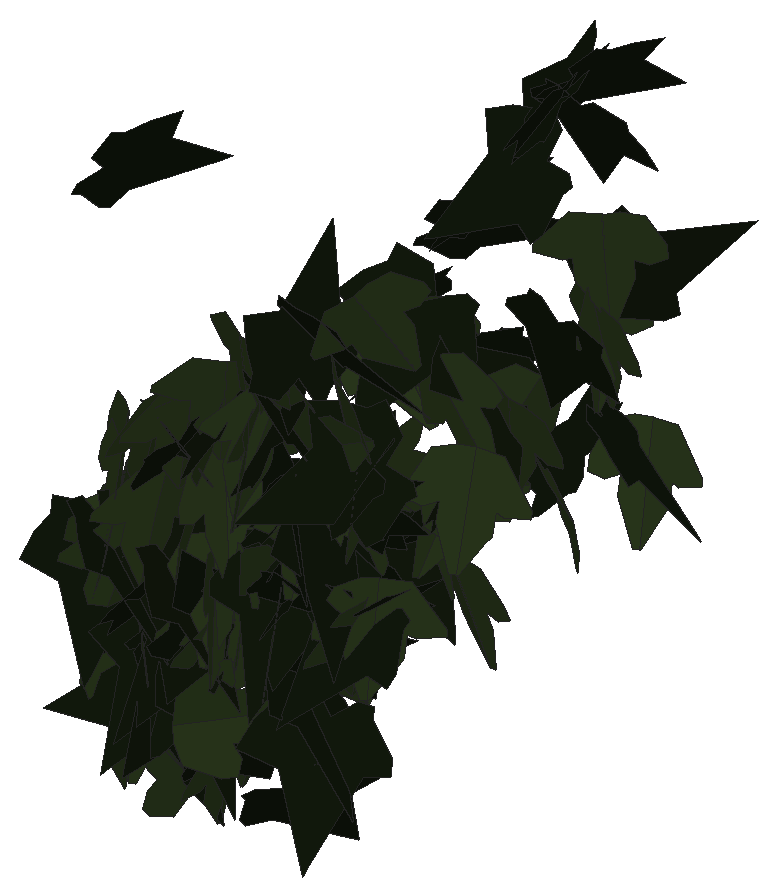
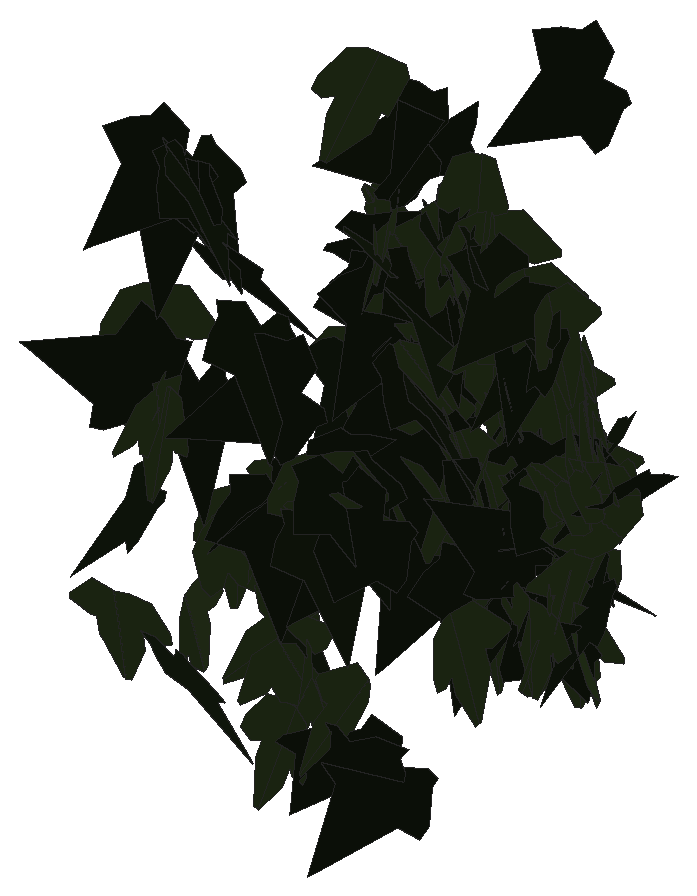
# SketchUp Ruby script. Lengths in inches.
U = 1.inch
M = Sketchup.active_model
def pt(a) = Geom::Point3d.new(a.map { |v| v * U })
def face(e, loops, mat)
  f = e.add_face(loops[0].map { |a| pt(a) })
  loops[1..].each { |l| e.add_face(l.map { |a| pt(a) }).erase! }
  f.material = f.back_material = mat if mat
  f
end
# faces: each face lists its corners as indices into pts; further lists are holes
def faces(e, pts, list, mat = nil) = list.each { |f| face(e, (f[0].is_a?(Array) ? f : [f]).map { |l| l.map { |i| pts[i] } }, mat) }
# xy, xz, yz: faces in a plane at the given z, y or x. An outline is a flat list of corners, or four numbers for a rectangle; further outlines are holes
def ring(l) = l.size == 4 ? [[l[0], l[1]], [l[2], l[1]], [l[2], l[3]], [l[0], l[3]]] : l.each_slice(2).to_a
def flat(e, list, mat, &to3) = list.each { |f| face(e, (f[0].is_a?(Array) ? f : [f]).map { |l| ring(l).map { |u, v| to3.(u, v) } }, mat) }
def xy(e, z, list, mat = nil) = flat(e, list, mat) { |x, y| [x, y, z] }
def xz(e, y, list, mat = nil) = flat(e, list, mat) { |x, z| [x, y, z] }
def yz(e, x, list, mat = nil) = flat(e, list, mat) { |y, z| [x, y, z] }
def lines(e, pts, list) = list.each { |a, b| e.add_line(pt(pts[a]), pt(pts[b])) }
# prism: a flat outline (further loops are holes) pulled along v
def prism(e, loops, v, mat = nil)
  f = face(e, loops, mat); d = Geom::Vector3d.new(v.map { |x| x * U })
  f.pushpull(f.normal.samedirection?(d) ? d.length : -d.length)
end
def box(e, o, s, mat = nil) = prism(e, [[o, [o[0] + s[0], o[1], o[2]], [o[0] + s[0], o[1] + s[1], o[2]], [o[0], o[1] + s[1], o[2]]]], [0, 0, s[2]], mat)
def at(x, y, z, deg = 0) = Geom::Transformation.translation(pt([x, y, z])) * Geom::Transformation.rotation(ORIGIN, Z_AXIS, deg.degrees)
def axes(o, x, y, z) = Geom::Transformation.new([*x, 0, *y, 0, *z, 0, *pt(o).to_a, 1])
def part(name) = M.definitions.add(name)
# library, detail: a bought-in or finely detailed component or shape, given as its bounding box
def library(name, o, s) = part(name).tap { |d| box(d.entities, o, s) }
def detail(e, o, s) = box(e.add_group.entities, o, s)
def put(e, d, t, mat = nil) = e.add_instance(d, t).tap { |i| i.material = mat if mat }
def group(e, t, mat = nil) = e.add_group.tap { |g| g.transformation = t; g.material = mat if mat }.entities
root = M.entities
M.materials.add("efeu1").color = [18, 25, 13]
M.materials.add("efeu2").color = [43, 57, 29]
c1 = part("ivyleaf_10")
p = [[0,0.5,-0.03],[-0.0625,2.02,-0.43],[-0.19,2.01,-0.46],[-0.54,1.05,-0.29],[-0.52,0.625,-0.18],[-0.83,0.76,-0.28],
  [-1.16,0.64,-0.33],[-1.15,0.33,-0.24],[-0.77,-0.39,0.02],[-0.3,-0.51,0.16],[0.04,-0.48,0.23],[-0.02,2.01,-0.4375],
  [-0.06,2.01,-0.43],[0.04,-0.49,0.23],[0.67,-0.49,0.14],[1.38,0.36,-0.2],[1.375,0.51,-0.24],[0.81,0.65,-0.19],
  [0.62,0.59,-0.15],[0.6,1.09,-0.28],[0.5,1.23,-0.31]]
faces(c1.entities,p,[[0,1,2,3,4,5,6,7,8,9,10],[11,12,0,13,14,15,16,17,18,19,20]],"efeu2")
c2 = part("ivyleaf_9")
p = [[1.54,2.16,1.25],[1.36,2.04,1.19],[-0.21,0.99,0.68],[-0.71,1.11,0.82],[-0.85,0.86,0.67],[-0.8,0.17,0.21],
  [-0.9,-0.01,0.1],[-0.67,-0.16,-0.02],[-0.08,-0.08,-0.05],[-0.03,-0.6,-0.4],[0.65,-0.88,-0.66],[0.83,-0.6,-0.49],
  [1.29,-0.42,-0.43],[1.8125,-0.07,-0.26],[1.21,0.44,0.15]]
faces(c2.entities,p,[[0,1,2,3,4,5,6,7,8,9,10,11,12,13,14]],"efeu1")
put(root,c1,axes([41.9,223.25,236.34],[-0.14655,-0.46971,0.08886],[0.0345,-0.10309,-0.48804],[0.47679,-0.13692,0.06263]))
put(root,c1,axes([43.12,223.04,238.36],[-0.46033,0.12611,0.14896],[-0.14145,0.04738,-0.47723],[-0.13448,-0.48151,-0.00795]))
put(root,c1,axes([43.13,223.35,237.54],[-0.13883,-0.43112,0.21181],[0.04974,-0.2322,-0.44001],[0.47776,-0.1011,0.10736]))
put(root,c2,axes([43.88,223.33,234.49],[-0.31378,-0.34921,-0.17204],[0.11314,0.12963,-0.46946],[0.37248,-0.33355,-0.00233]))
put(root,c1,axes([41.27,223.24,235.78],[0.33453,-0.37126,0.0158],[0.02306,-0.00048,-0.49947],[0.37088,0.33491,0.0168]))
put(root,c2,axes([44.39,223.45,237.38],[-0.39107,-0.1524,0.27174],[-0.23964,-0.13155,-0.41865],[0.1991,-0.45768,0.02985]))
put(root,c2,axes([42.32,223.33,235.05],[-0.4867,-0.03334,-0.1096],[0.11067,-0.0132,-0.48742],[0.02961,-0.49871,0.02023]))
put(root,c2,axes([43.23,223.33,237.06],[-0.08331,-0.00209,-0.49301],[0.49276,-0.01636,-0.0832],[-0.01578,-0.49973,0.00479]))
put(root,c1,axes([42.57,223.3125,235.58],[-0.09073,0.40705,-0.27582],[0.05377,-0.27058,-0.41701],[-0.48875,-0.10533,0.00532]))
put(root,c2,axes([41.67,222.79,239.95],[0.25473,0.28777,0.31984],[0.21646,0.23551,-0.38429],[-0.37183,0.33425,-0.0046]))
put(root,c2,axes([43.83,223.43,236.4375],[0.06562,-0.48821,0.08567],[-0.0004,-0.08647,-0.49247],[0.49567,0.06457,-0.01174]))
put(root,c2,axes([43.4,223.39,235.9],[-0.38034,-0.27863,-0.16646],[0.1632,0.05748,-0.46911],[0.28055,-0.41117,0.04722]))
put(root,c1,axes([42.75,223.2,237.87],[-0.37516,-0.32831,0.03826],[-0.03439,-0.01878,-0.49846],[0.32874,-0.37664,-0.00849]))
put(root,c2,axes([41.2,223.29,235.71],[0.29546,-0.40334,-0.00453],[0.00177,0.00691,-0.49995],[0.40336,0.29542,0.00551]))
put(root,c1,axes([42.85,223.45,237.29],[0.25653,-0.28307,0.32259],[0.2162,-0.23943,-0.38201],[0.37075,0.33548,-0.00045]))
put(root,c2,axes([42.14,223.29,234.29],[-0.42513,0.12072,0.23386],[-0.24322,-0.01049,-0.43673],[-0.10054,-0.4851,0.06764]))
put(root,c1,axes([41.86,223.26,237.22],[0.04929,-0.49756,0.00001],[-0.00013,-0.00003,-0.5],[0.49756,0.04929,-0.00013]))
put(root,c1,axes([42.54,223.28,235.76],[0.49119,-0.06142,0.07044],[0.06923,-0.01408,-0.49498],[0.06278,0.49601,-0.00533]))
put(root,c2,axes([44.35,223.38,235.83],[-0.49168,-0.07529,-0.05078],[0.05089,0.00312,-0.49739],[0.07521,-0.49429,0.00459]))
put(root,c1,axes([44.15,223.48,237.24],[-0.09405,0.23419,-0.43163],[0.11552,-0.4166,-0.2512],[-0.47729,-0.14698,0.02426]))
put(root,c2,axes([41.78,223.6,234.07],[0.1439,-0.14496,-0.45638],[0.32512,-0.32029,0.20424],[-0.35156,-0.35553,0.00208]))
put(root,c2,axes([43.2,223.18,237.88],[0.4379,-0.23619,-0.04961],[-0.04004,0.03024,-0.49748],[0.23799,0.43966,0.00757]))
put(root,c1,axes([42.23,223.27,237.38],[-0.15829,-0.47427,-0.0041],[0.01044,0.00084,-0.49989],[0.47417,-0.15834,0.00964]))
put(root,c2,axes([42.84,223.1,237.58],[-0.2834,0.40684,0.06454],[-0.0429,0.04876,-0.49576],[-0.40969,-0.28653,0.00726]))
put(root,c2,axes([41.94,223.56,234.54],[-0.30019,-0.38956,0.09017],[-0.05344,-0.07266,-0.4918],[0.39627,-0.3049,0.00199]))
put(root,c1,axes([42.6875,222.89,234.24],[-0.00004,0.01216,0.49985],[0.131,0.48239,-0.01172],[-0.48253,0.13096,-0.00323]))
put(root,c2,axes([42.04,223.35,235.46],[0.2615,-0.42615,-0.00415],[0.0243,0.01977,-0.49902],[0.42547,0.26078,0.03105]))
put(root,c1,axes([41.32,223.34,236.53],[0.33725,-0.36605,0.04761],[0.06246,-0.00698,-0.49603],[0.36381,0.34053,0.04102]))
put(root,c1,axes([41.43,223.4,235.5625],[-0.17036,-0.44687,0.14588],[-0.01752,-0.14903,-0.47695],[0.46976,-0.16762,0.03512]))
put(root,c2,axes([43.49,223.41,234.8],[0.23339,-0.44121,0.02939],[0.02254,-0.02132,-0.49904],[0.44161,0.23426,0.00994]))
put(root,c2,axes([40.99,223.52,235.39],[-0.08743,-0.49224,0.00783],[0.00955,-0.00964,-0.49982],[0.4922,-0.08724,0.01109]))
put(root,c2,axes([43.65,223.26,238.7],[0.42423,-0.16786,0.20457],[0.20345,-0.04027,-0.45496],[0.16922,0.46925,0.03413]))
put(root,c1,axes([44.27,223.31,235.78],[-0.02645,-0.49573,-0.0596],[0.00143,0.05961,-0.49643],[0.4993,-0.02643,-0.00174]))
put(root,c1,axes([41.56,223.42,234.4],[-0.22596,0.36232,-0.26013],[0.09052,-0.24828,-0.42445],[-0.43675,-0.23891,0.04661]))
put(root,c1,axes([43.14,223.43,235.54],[0.3405,-0.3398,0.13637],[0.12332,-0.06892,-0.47963],[0.34475,0.36026,0.03687]))
put(root,c1,axes([41.4,223.3,236.77],[0.31898,-0.37987,-0.06287],[0.02555,0.10235,-0.48875],[0.38419,0.30859,0.08471]))
put(root,c1,axes([42.98,223.42,237.47],[0.19634,-0.45494,0.06692],[0.0306,-0.05968,-0.49548],[0.45882,0.19866,0.00441]))
put(root,c2,axes([43.72,223.14,235.91],[0.37237,0.25349,-0.21699],[-0.19378,-0.10042,-0.44985],[-0.27164,0.41912,0.02346]))
put(root,c2,axes([44.29,223.4,237.34],[-0.44378,0.22708,0.03866],[-0.0813,-0.0759,-0.48747],[-0.21552,-0.43895,0.10428]))
put(root,c1,axes([43.67,223.39,237.33],[-0.26865,-0.01037,0.42157],[0.4217,-0.0065,0.26857],[-0.00009,0.49985,0.01224]))
put(root,c2,axes([43.68,223.14,238.3],[-0.19276,-0.2182,0.40649],[0.26951,0.3043,0.29115],[-0.37445,0.33135,0.00031]))
put(root,c1,axes([42.22,223.52,236.48],[0.23289,-0.40959,0.16734],[0.08387,-0.1448,-0.47117],[0.43443,0.24753,0.00126]))
put(root,c1,axes([44.46,223.3,235.98],[0.39356,0.30755,-0.02288],[-0.08415,0.0714,-0.48767],[-0.2967,0.3877,0.10796]))
put(root,c1,axes([42.49,223.49,234.92],[0.04805,-0.48298,0.1201],[-0.00352,-0.12099,-0.48513],[0.49767,0.04577,-0.01502]))
put(root,c1,axes([44.43,223.2,239.22],[-0.2698,-0.33894,-0.24966],[0.15713,0.19402,-0.43321],[0.39054,-0.31221,0.00183]))
put(root,c2,axes([42.375,223.53,234.82],[0.2645,0.19211,0.37833],[-0.30001,-0.2306,0.32683],[0.30006,-0.3999,-0.00672]))
put(root,c1,axes([43.71,223.4,236.81],[0.32683,0.35631,-0.12737],[-0.11332,-0.06841,-0.48216],[-0.36102,0.34404,0.03604]))
put(root,c1,axes([42.48,223.46,236.87],[0.06764,-0.49038,-0.07039],[0.00861,-0.06987,0.49502],[-0.49533,-0.06818,-0.00101]))
put(root,c2,axes([43.57,223.21,237.14],[-0.09879,0.48624,-0.06175],[0.00797,-0.06139,-0.49615],[-0.49008,-0.09902,0.00438]))
put(root,c2,axes([43.39,223.0625,237.42],[-0.11851,0.3672,0.31799],[-0.13461,0.28967,-0.38467],[-0.46673,-0.17679,0.0302]))
put(root,c1,axes([42.625,223.35,236.72],[0.18509,0.46379,-0.02524],[-0.01383,-0.02165,-0.49934],[-0.46427,0.18555,0.00481]))
put(root,c2,axes([41.97,223.25,237.02],[0.47347,-0.10855,-0.1185],[-0.11332,0.03589,-0.48566],[0.11395,0.48675,0.00939]))
put(root,c1,axes([41.14,223.48,235.42],[0.19253,-0.4498,-0.10303],[0.03337,-0.09777,0.48921],[-0.46024,-0.19525,-0.00763]))
put(root,c2,axes([42.1,223.5625,234.28],[0.18573,-0.46135,0.05161],[0.02487,-0.04562,-0.49729],[0.46356,0.18729,0.006]))
put(root,c1,axes([42.87,223.41,235.18],[0.4282,-0.18609,-0.17893],[-0.15719,0.08696,-0.46661],[0.20479,0.45586,0.01597]))
put(root,c2,axes([41.81,223.4375,235.27],[-0.1729,0.40011,-0.24499],[0.03605,-0.24899,-0.43209],[-0.46777,-0.16708,0.05725]))
put(root,c2,axes([42.26,223.15,237.05],[0.07168,0.48972,0.07096],[0.02076,0.06866,-0.49483],[-0.4944,0.07388,-0.01049]))
put(root,c2,axes([43.55,223.15,233.73],[0.29498,0.40204,0.03677],[0.01708,0.03307,-0.49861],[-0.40336,0.29541,0.00577]))
put(root,c1,axes([42.54,223.51,235.11],[-0.2824,-0.4106,0.04075],[0.02622,-0.06714,-0.49478],[0.41178,-0.27731,0.05945]))
put(root,c2,axes([41.67,223.55,235.83],[-0.24359,-0.34324,-0.26991],[0.15629,0.22006,-0.42089],[0.40772,-0.28942,0.00008]))
put(root,c1,axes([42.6,223.53,235.13],[0.35754,-0.34698,0.04202],[0.06931,0.01147,-0.49504],[0.34258,0.35982,0.0563]))
put(root,c1,axes([41.82,223.64,233.11],[-0.15676,0.37448,0.29187],[0.11163,-0.26968,0.40597],[0.46148,0.19244,0.00095]))
put(root,c1,axes([41.06,223.69,233.33],[0.20336,-0.29877,-0.34552],[0.19805,-0.28314,0.3614],[-0.41161,-0.28385,0.00318]))
put(root,c1,axes([44.03,223.375,238.02],[-0.37913,0.30588,0.11268],[-0.10033,0.05495,-0.48674],[-0.31016,-0.39168,0.01971]))
put(root,c1,axes([41.21,223.63,235.3],[0.18691,-0.4444,-0.13258],[0.04584,-0.12453,0.48207],[-0.46148,-0.19236,-0.00581]))
put(root,c1,axes([42.51,223.53,233.7],[0.05718,-0.49209,-0.06766],[-0.00177,0.0679,-0.49536],[0.49672,0.05689,0.00602]))
put(root,c1,axes([41.65,223.42,234.24],[0.11582,-0.43804,-0.21144],[-0.0073,0.21576,-0.45099],[0.48635,0.10755,0.04358]))
put(root,c1,axes([43.7,223.62,236.35],[-0.41779,-0.23762,0.13779],[-0.08737,-0.12283,-0.47674],[0.26042,-0.42243,0.06112]))
put(root,c2,axes([43.5,223.21,236.73],[-0.00777,0.40839,0.28837],[-0.13459,0.27605,-0.39457],[-0.48148,-0.08375,0.10564]))
put(root,c1,axes([43.18,223.44,235.76],[-0.09339,-0.43376,0.23051],[0.04395,0.22631,0.44368],[-0.48923,0.10313,-0.00414]))
put(root,c2,axes([43.95,223.36,236.88],[0.35952,0.30266,-0.1707],[-0.15103,-0.08511,-0.46898],[-0.31294,0.38878,0.03022]))
put(root,c2,axes([43.47,223.38,235.89],[-0.25879,0.40535,0.13684],[-0.07364,0.11534,-0.48091],[-0.42144,-0.26906,0]))
put(root,c1,axes([41.21,223.57,235.65],[0.42196,0.26495,0.04189],[0.02927,0.03214,-0.49811],[-0.26664,0.42281,0.01162]))
put(root,c1,axes([41.33,223.66,233.86],[-0.49768,-0.02819,0.03899],[-0.02872,-0.15096,-0.4758],[0.0386,-0.47583,0.14864]))
put(root,c1,axes([41.27,223.46,234.47],[0.13035,0.46217,0.13932],[-0.01431,0.14795,-0.4774],[-0.4825,0.12047,0.0518]))
put(root,c1,axes([41.05,223.47,235.11],[-0.2198,-0.26989,0.35895],[0.22377,0.28068,0.34806],[-0.38938,0.31365,-0.0026]))
put(root,c1,axes([42.74,223.67,235.42],[-0.413,-0.00089,0.28183],[-0.2741,-0.11505,-0.40204],[0.06557,-0.48658,0.09455]))
put(root,c2,axes([43.48,223.68,236.31],[-0.24394,0.37324,-0.22625],[0.09788,-0.2058,-0.44505],[-0.42534,-0.26142,0.02733]))
put(root,c2,axes([43.76,223.38,235.17],[0.26419,0.42444,0.00717],[-0.03262,0.02872,-0.49811],[-0.42325,0.26272,0.04287]))
put(root,c2,axes([42.25,223.29,237.49],[0.27337,0.35792,0.21716],[-0.01385,0.26695,-0.42255],[-0.41842,0.22501,0.15586]))
put(root,c2,axes([41.01,223.58,234.38],[0.41896,-0.13111,-0.23934],[-0.22609,0.07882,-0.43894],[0.15283,0.47602,0.00676]))
put(root,c2,axes([43.82,223.41,236.78],[0.28145,0.40536,0.08046],[0.05587,0.05913,-0.49334],[-0.40947,0.28669,-0.01201]))
put(root,c2,axes([44.21,223.33,235.72],[0.25039,0.38241,0.20264],[0.00392,0.2321,-0.44285],[-0.43277,0.22336,0.11323]))
put(root,c2,axes([41.46,223.74,233.85],[-0.15319,-0.08307,-0.46865],[0.40416,0.23732,-0.17417],[0.25138,-0.43218,-0.00557]))
put(root,c2,axes([42.63,223.51,233.83],[0.13267,0.48102,0.03185],[0.00719,0.03106,-0.49898],[-0.48202,0.13286,0.00132]))
put(root,c2,axes([41.9375,223.59,234.37],[-0.06285,-0.02436,0.49544],[0.4707,0.15462,0.06732],[-0.15649,0.47487,0.00349]))
put(root,c1,axes([41.66,223.86,233.92],[0.4771,-0.13665,0.06082],[0.08084,0.06453,-0.48918],[0.12584,0.47662,0.08367]))
put(root,c2,axes([43.43,223.77,235.76],[0.14227,0.43897,-0.19252],[-0.0855,-0.17436,-0.46075],[-0.47165,0.16402,0.02545]))
put(root,c1,axes([43.05,224,234.93],[-0.21951,0.01381,-0.44902],[0.4128,-0.19095,-0.20768],[-0.17722,-0.46189,0.07243]))
put(root,c1,axes([42.25,224.41,233.72],[-0.01355,-0.49697,0.05327],[0.00012,-0.05329,-0.49715],[0.49982,-0.01346,0.00156]))
put(root,c1,axes([43.12,226.39,235.5625],[0.48284,0.12907,-0.01437],[-0.01977,0.01838,-0.49927],[-0.12835,0.4827,0.02286]))
put(root,c2,axes([42.32,226.83,236.95],[-0.31124,-0.38552,0.06715],[-0.05246,-0.04392,-0.4953],[0.38779,-0.31535,-0.01311]))
put(root,c1,axes([42.66,226.65,236.28],[-0.39268,0.07428,-0.30047],[0.27469,-0.14006,-0.39361],[-0.14264,-0.4742,0.06919]))
put(root,c2,axes([43.68,226.79,238.9375],[-0.49015,0.05756,0.08025],[-0.07968,0.00953,-0.49352],[-0.05834,-0.49658,-0.00017]))
put(root,c2,axes([43.98,226.71,239.86],[-0.1848,0.44597,-0.13021],[0.04018,-0.12426,-0.48264],[-0.46285,-0.18885,0.01009]))
put(root,c1,axes([42.17,226.83,236.75],[-0.37433,-0.33132,0.01019],[-0.00918,-0.00499,-0.49989],[0.33135,-0.37443,-0.00235]))
put(root,c2,axes([41.89,226.8,236.81],[-0.08486,0.46744,-0.15589],[-0.04373,-0.16471,-0.47006],[-0.4908,-0.06615,0.06884]))
put(root,c2,axes([43.86,226.81,237.23],[0.31224,0.12567,-0.36975],[-0.34854,-0.12386,-0.33642],[-0.17615,0.46783,0.01025]))
put(root,c1,axes([41.73,226.85,236.39],[0.31916,0.2921,0.25063],[0.19653,0.15625,-0.43239],[-0.33092,0.37452,-0.01508]))
put(root,c2,axes([42.62,226.97,235.26],[-0.36582,0.33156,-0.07901],[0.06077,-0.05061,-0.49371],[-0.33538,-0.37082,-0.00327]))
put(root,c2,axes([42.6875,227.2,236.38],[0.09498,-0.4908,-0.00977],[0.03805,0.01729,-0.49825],[0.48942,0.0939,0.04064]))
put(root,c1,axes([43.23,226.94,236],[-0.47794,0.06373,0.13235],[-0.1301,0.02546,-0.4821],[-0.06819,-0.49527,-0.00776]))
put(root,c2,axes([44.12,226.85,239.65],[0.35646,0.19729,-0.28985],[-0.29022,-0.06592,-0.40178],[-0.19675,0.45468,0.06752]))
put(root,c2,axes([43.9,226.78,239.68],[-0.17093,0.3935,0.25679],[-0.12774,0.22405,-0.42835],[-0.45218,-0.21204,0.02394]))
put(root,c1,axes([43.04,227.34,235.96],[-0.1507,-0.37356,0.29622],[-0.04091,-0.29939,-0.39836],[0.47499,-0.1443,0.05967]))
put(root,c1,axes([44.18,227.11,238.22],[-0.41153,-0.28383,-0.00909],[0.03418,-0.03362,-0.4977],[0.28191,-0.41026,0.04708]))
put(root,c2,axes([42.94,226.9,238.26],[-0.04119,0.49814,0.01271],[-0.0167,0.01137,-0.49959],[-0.49802,-0.04158,0.0157]))
put(root,c2,axes([41.36,226.89,236.5],[0.46258,0.18856,0.02163],[0.01959,0.00925,-0.49953],[-0.18878,0.46299,0.00117]))
put(root,c1,axes([41.9,227.33,234.52],[0.28983,-0.23158,0.33522],[0.33997,-0.08926,-0.3556],[0.22454,0.43406,0.10573]))
put(root,c1,axes([42.29,227.3125,234.8125],[0.16326,0.41289,-0.22992],[-0.15897,-0.1811,-0.4381],[-0.44505,0.21615,0.07214]))
put(root,c2,axes([42.53,227.05,236.39],[0.16116,0.45021,-0.14608],[-0.07102,-0.12957,-0.47767],[-0.46795,0.17472,0.02219]))
put(root,c2,axes([44.05,226.89,239.94],[0.29323,0.33512,0.2274],[0.11687,0.19879,-0.44365],[-0.38776,0.31333,0.03825]))
put(root,c2,axes([41.92,227.04,236.15],[-0.05197,0.4952,0.04555],[-0.09204,0.03543,-0.49018],[-0.4887,-0.05933,0.08748]))
put(root,c2,axes([42.42,226.97,237.73],[0.35425,0.1599,0.31454],[0.25292,0.19571,-0.38435],[-0.24604,0.43143,0.05778]))
put(root,c1,axes([42.35,227.25,233.83],[-0.45929,0.18866,-0.05884],[0.05683,-0.01651,-0.49649],[-0.18927,-0.46275,-0.00628]))
put(root,c1,axes([43.99,227.38,237.27],[-0.01032,0.47765,-0.14745],[-0.0307,-0.14781,-0.47666],[-0.49895,-0.00078,0.03238]))
put(root,c1,axes([42.42,226.95,234.92],[0.07626,0.12306,0.47858],[0.00302,0.48412,-0.12496],[-0.49414,0.02195,0.0731]))
put(root,c2,axes([44.11,227.25,236.08],[0.42044,-0.24498,-0.11495],[-0.07138,0.10448,-0.48372],[0.26103,0.42316,0.05288]))
put(root,c2,axes([41.01,227.03,233.6875],[0.34439,0.34315,0.1168],[0.07818,0.08701,-0.48612],[-0.35395,0.3531,0.00628]))
put(root,c1,axes([43.96,227.29,237.125],[-0.46127,0.18344,0.05986],[-0.06359,0.00192,-0.49594],[-0.18217,-0.46513,0.02156]))
put(root,c2,axes([41.27,227.5,234.11],[-0.10243,-0.31069,-0.37813],[0.21755,0.31715,-0.31952],[0.43839,-0.22997,0.07021]))
put(root,c1,axes([43.51,227.32,234.875],[0.16656,0.04319,-0.46946],[-0.27081,0.41632,-0.05778],[0.3859,0.27352,0.16207]))
put(root,c1,axes([41.42,227.27,234.53],[-0.03316,0.24462,0.43481],[-0.11287,0.4208,-0.24534],[-0.48596,-0.11442,0.02731]))
put(root,c2,axes([44.0625,227.42,237.5],[0.06454,0.03924,0.49426],[0.47315,0.1441,-0.07322],[-0.14819,0.47718,-0.01854]))
put(root,c1,axes([43.74,228.28,235.27],[0.49536,0.04299,0.05268],[0.05286,0.00017,-0.4972],[-0.04277,0.49815,-0.00438]))
put(root,c2,axes([42.95,228.28,234.87],[-0.29315,0.36235,0.18102],[-0.17132,0.09156,-0.46072],[-0.36703,-0.33214,0.07048]))
